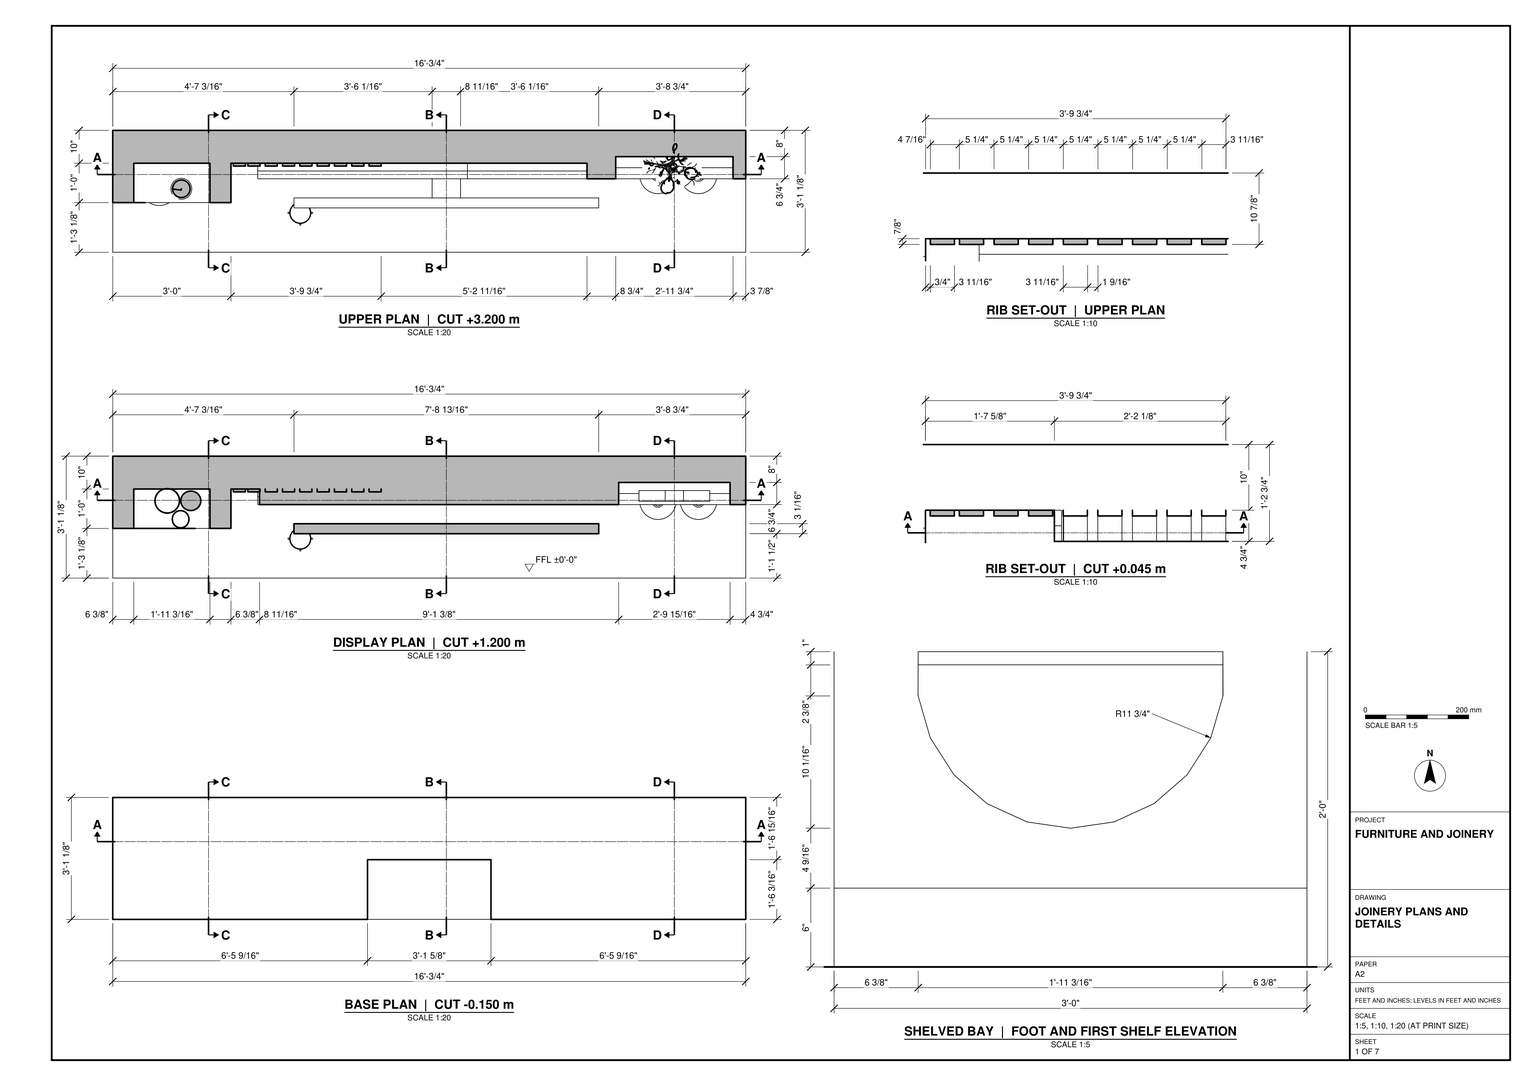
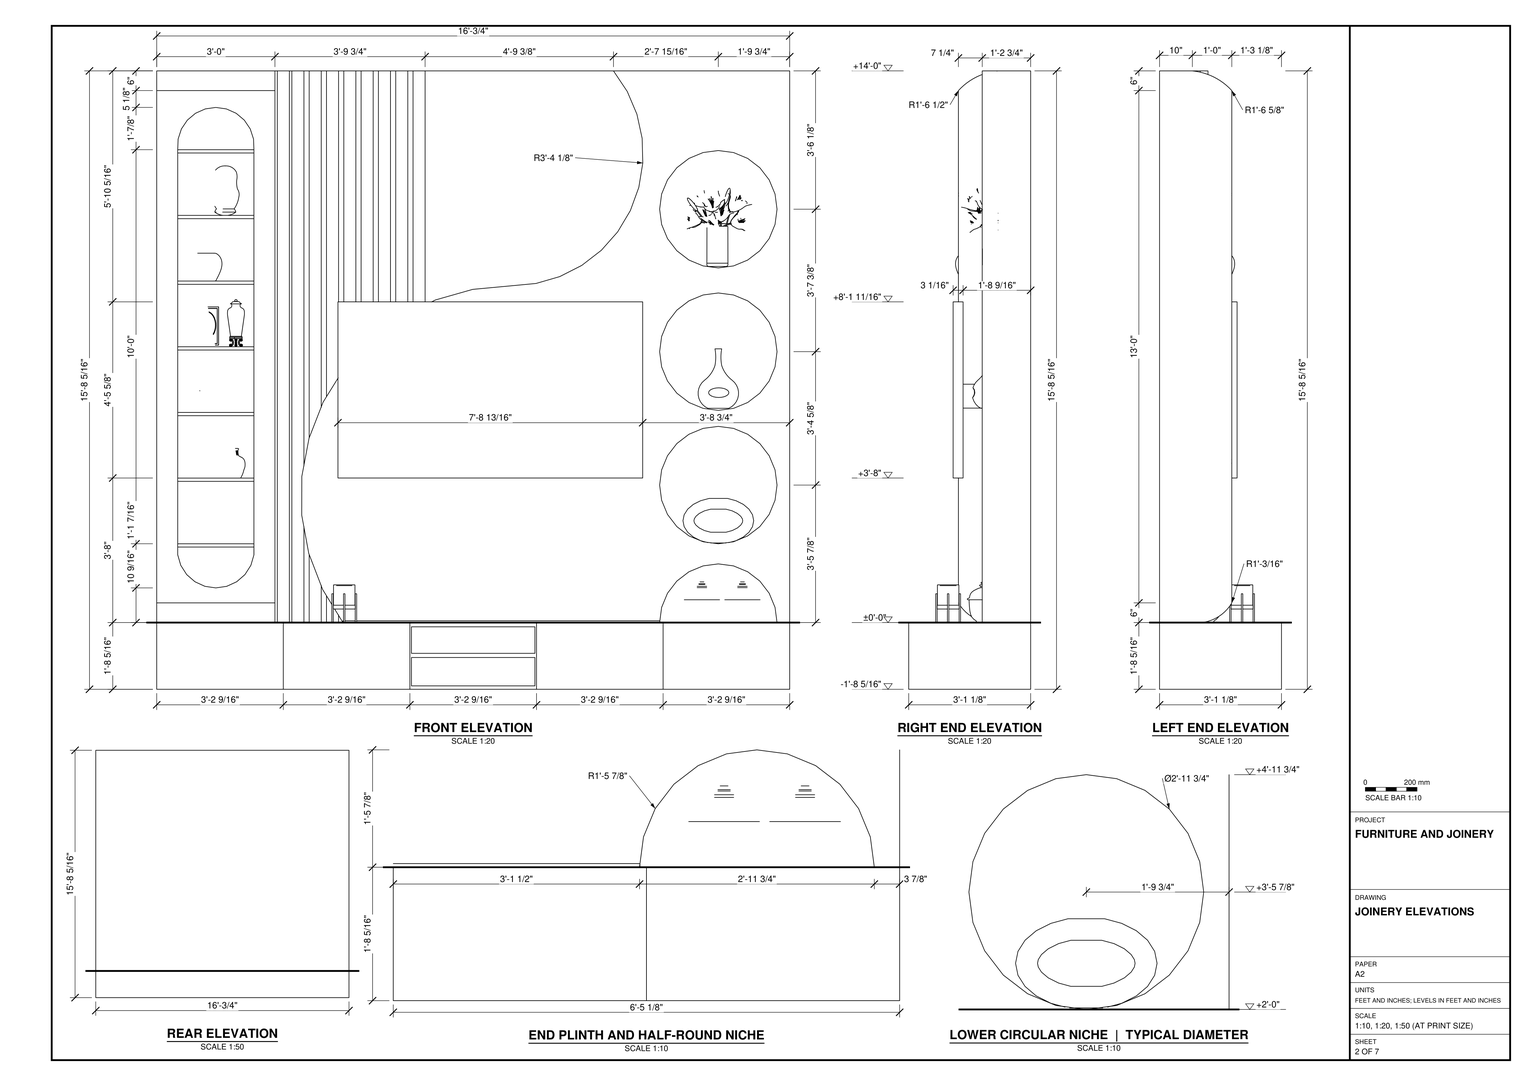
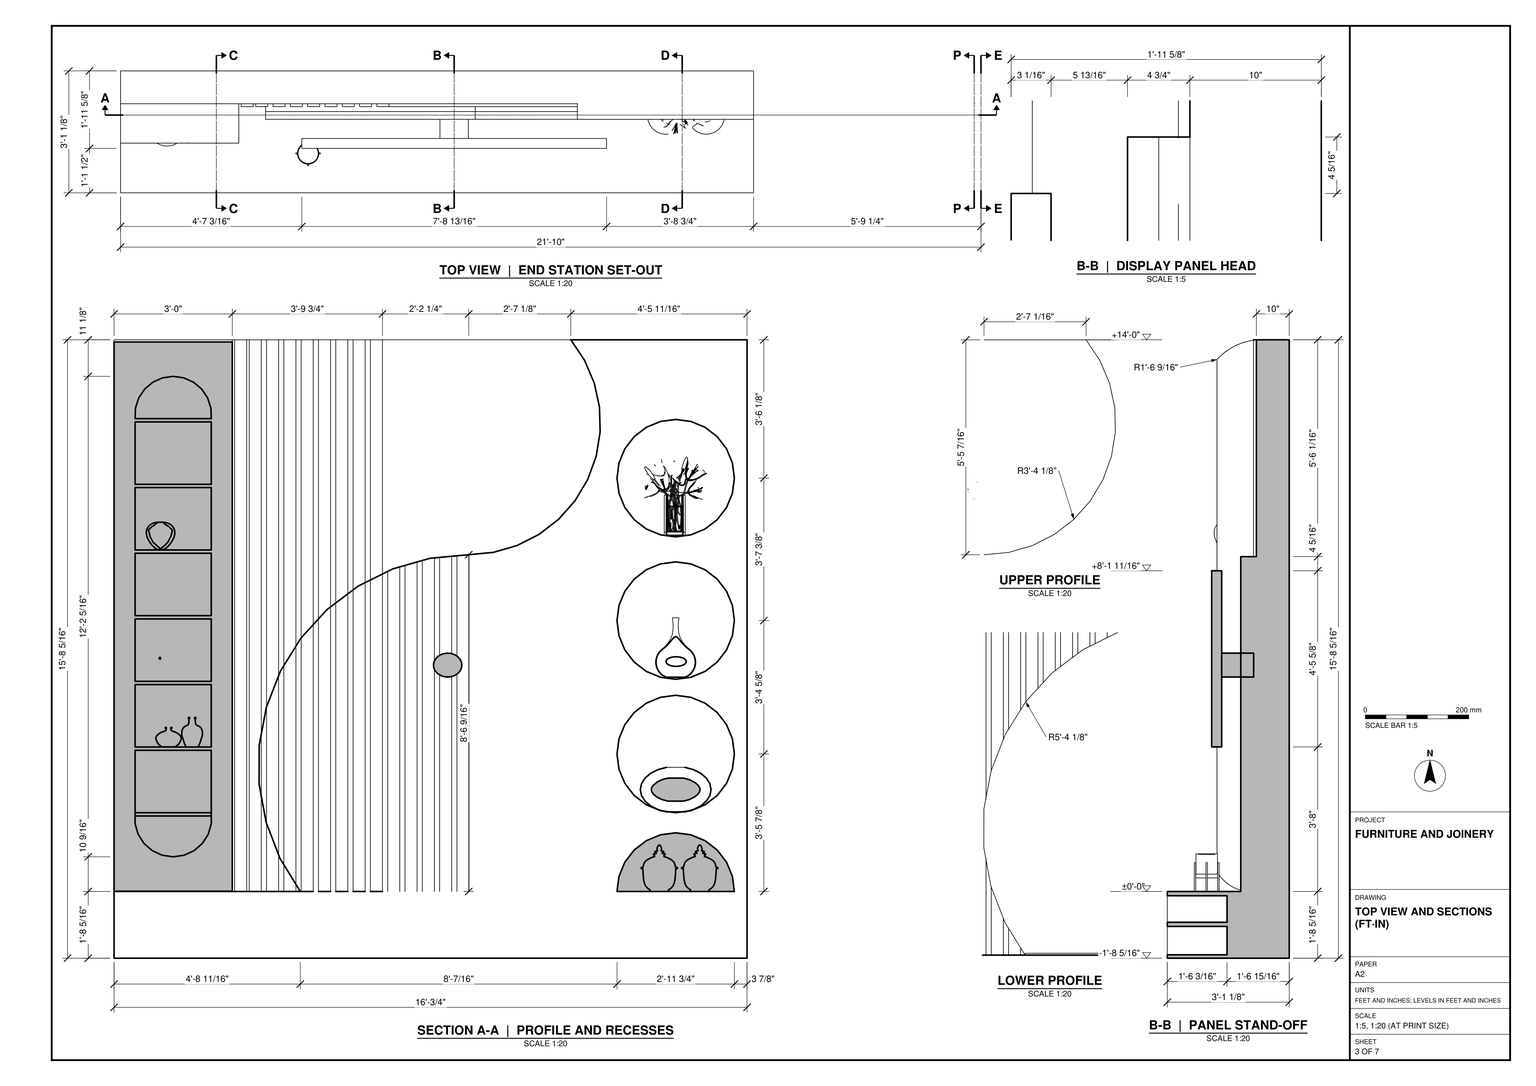
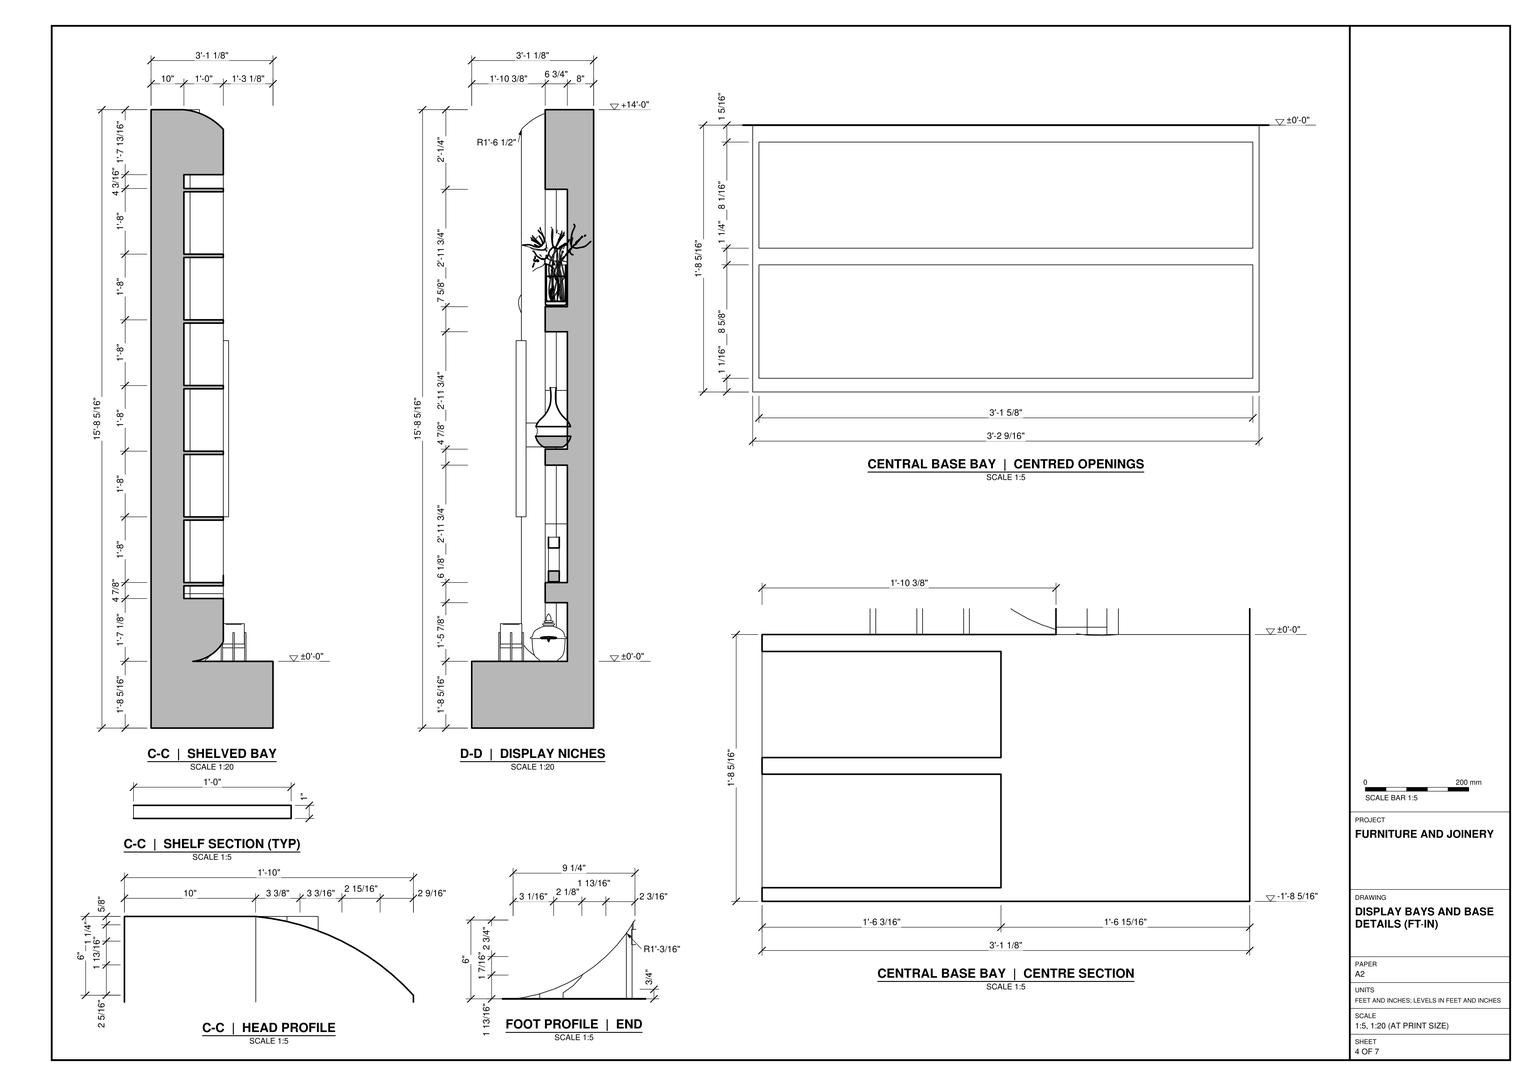
Build the display wall in SketchUp from task_files/diagram_01.pdf. Work in feet and inches. Follow the top-view end-station set-out: the overall span is 21'-10", but the joinery body itself is 16'-3/4" wide. The overall depth is 3'-1 1/8" and the overall height is 15'-8 5/16". Use ±0'-0" as the datum at the top of the plinth, with the base at -1'-8 5/16" and the wall head at +14'-0".

Form the plinth with the central setback shown in plan and the two stacked fronts shown in elevation. At the left, build the tall shelved bay with rounded ends to its opening. Beside it, model the individual vertical ribs, following the rib set-out in plan and the sweeping boundary between the ribbed and smooth faces in section A-A. Mount the rectangular display panel in front of this surface, leaving the stand-off visible in section B-B. At the right, form three circular display recesses above a half-round recess that meets the plinth. Follow the plans and sections for recess depths, backing thicknesses and end profiles.

Decor and loose items in the shelves and niches may be any suitable library components. Keep the joinery pieces in separate groups or components and use components for repeated parts. Save one SketchUp model as output_files/ribbed_display_wall_with_shelving_and_recessed_niches.skp.

# SketchUp Ruby script. Lengths in inches.
U = 1.inch
M = Sketchup.active_model
def pt(a) = Geom::Point3d.new(a.map { |v| v * U })
def face(e, loops, mat)
  f = e.add_face(loops[0].map { |a| pt(a) })
  loops[1..].each { |l| e.add_face(l.map { |a| pt(a) }).erase! }
  f.material = f.back_material = mat if mat
  f
end
# faces: each face lists its corners as indices into pts; further lists are holes
def faces(e, pts, list, mat = nil) = list.each { |f| face(e, (f[0].is_a?(Array) ? f : [f]).map { |l| l.map { |i| pts[i] } }, mat) }
# xy, xz, yz: faces in a plane at the given z, y or x. An outline is a flat list of corners, or four numbers for a rectangle; further outlines are holes
def ring(l) = l.size == 4 ? [[l[0], l[1]], [l[2], l[1]], [l[2], l[3]], [l[0], l[3]]] : l.each_slice(2).to_a
def flat(e, list, mat, &to3) = list.each { |f| face(e, (f[0].is_a?(Array) ? f : [f]).map { |l| ring(l).map { |u, v| to3.(u, v) } }, mat) }
def xy(e, z, list, mat = nil) = flat(e, list, mat) { |x, y| [x, y, z] }
def xz(e, y, list, mat = nil) = flat(e, list, mat) { |x, z| [x, y, z] }
def yz(e, x, list, mat = nil) = flat(e, list, mat) { |y, z| [x, y, z] }
def lines(e, pts, list) = list.each { |a, b| e.add_line(pt(pts[a]), pt(pts[b])) }
# prism: a flat outline (further loops are holes) pulled along v
def prism(e, loops, v, mat = nil)
  f = face(e, loops, mat); d = Geom::Vector3d.new(v.map { |x| x * U })
  f.pushpull(f.normal.samedirection?(d) ? d.length : -d.length)
end
def box(e, o, s, mat = nil) = prism(e, [[o, [o[0] + s[0], o[1], o[2]], [o[0] + s[0], o[1] + s[1], o[2]], [o[0], o[1] + s[1], o[2]]]], [0, 0, s[2]], mat)
def at(x, y, z, deg = 0) = Geom::Transformation.translation(pt([x, y, z])) * Geom::Transformation.rotation(ORIGIN, Z_AXIS, deg.degrees)
def axes(o, x, y, z) = Geom::Transformation.new([*x, 0, *y, 0, *z, 0, *pt(o).to_a, 1])
def part(name) = M.definitions.add(name)
# library, detail: a bought-in or finely detailed component or shape, given as its bounding box
def library(name, o, s) = part(name).tap { |d| box(d.entities, o, s) }
def detail(e, o, s) = box(e.add_group.entities, o, s)
def put(e, d, t, mat = nil) = e.add_instance(d, t).tap { |i| i.material = mat if mat }
def group(e, t, mat = nil) = e.add_group.tap { |g| g.transformation = t; g.material = mat if mat }.entities
root = M.entities
M.materials.add("CUEVE TILE").color = [204, 198, 186]
M.materials.add("Emissive").color = [255, 255, 255]
M.materials.add("NETFLEX TEXTURE").color = [73, 67, 67]
M.materials.add("WALL TILE").color = [226, 214, 203]
M.materials.add("WHITE WOOD TEXTURE FOR CABIN").color = [208, 209, 205]
M.materials.add("WOOD TEXTURE").color = [111, 66, 36]
M.materials.add("[Leather Red Brown]").color = [76, 40, 8]
M.materials.add("[Slate Light Tile]").color = [54, 54, 54]
c1 = library("skp5FE5",[-20.25,-9.09,-9.95],[33.36,28.86,33.4])
c2 = library("skp86D6",[-3.15,-10.14,-7.26],[20.14,20.18,14.98])
c3 = library("Lidded urn",[0,0,0],[20.74,20.74,57.81])
c4 = library("Lily Flower",[-11.23,-7.61,-0.93],[19.43,20.89,23.03])
c5 = library("KARE 65351 Vase Hole Alu Bottle ( Vase Hole Alu Bottle )",[-6.15,-1.29,0],[12.3,2.58,18.11])
c6 = part("KARE 64859 Vase Hole Alu Length ( Vase Hole Alu Quer )")
xy(c6.entities,0.2,[[-2.34,0,2.34,2.76]])
xy(c6.entities,2.96,[[-1.98,0,1.98,2.76]])
xy(c6.entities,8.85,[[-1.98,0,1.98,2.76]])
xz(c6.entities,0,[[[-2.34,0.2,2.34,0.2,4.53,0.79,6.4,1.73,7.84,2.95,8.75,4.38,9.06,5.91,8.75,7.43,7.84,8.86,6.4,10.08,4.53,11.02,2.34,11.61,-2.34,11.61,-4.53,11.02,-6.4,10.08,-7.84,8.86,-8.75,7.43,-9.06,5.91,-8.75,4.38,-7.84,2.95,-6.4,1.73,-4.53,0.79],[-1.98,2.96,-3.54,3.38,-4.87,4.05,-5.74,4.78,-6.15,5.42,-6.24,5.91,-6.15,6.39,-5.74,7.03,-4.87,7.77,-3.54,8.43,-1.98,8.85,1.98,8.85,3.54,8.43,4.87,7.77,5.74,7.03,6.15,6.39,6.24,5.91,6.15,5.42,5.74,4.78,4.87,4.05,3.54,3.38,1.98,2.96]]])
xz(c6.entities,2.76,[[[-2.34,0.2,-4.53,0.79,-6.4,1.73,-7.84,2.95,-8.75,4.38,-9.06,5.91,-8.75,7.43,-7.84,8.86,-6.4,10.08,-4.53,11.02,-2.34,11.61,2.34,11.61,4.53,11.02,6.4,10.08,7.84,8.86,8.75,7.43,9.06,5.91,8.75,4.38,7.84,2.95,6.4,1.73,4.53,0.79,2.34,0.2],[-1.98,2.96,1.98,2.96,3.54,3.38,4.87,4.05,5.74,4.78,6.15,5.42,6.24,5.91,6.15,6.39,5.74,7.03,4.87,7.77,3.54,8.43,1.98,8.85,-1.98,8.85,-3.54,8.43,-4.87,7.77,-5.74,7.03,-6.15,6.39,-6.24,5.91,-6.15,5.42,-5.74,4.78,-4.87,4.05,-3.54,3.38]]])
p = [[-2.34,0,0.2],[-4.53,0,0.79],[-4.53,2.76,0.79],[-2.34,2.76,0.2],[4.53,0,0.79],[2.34,0,0.2],
  [2.34,2.76,0.2],[4.53,2.76,0.79],[-6.4,0,1.73],[-6.4,2.76,1.73],[6.4,0,1.73],[6.4,2.76,1.73],
  [-7.84,0,2.95],[-7.84,2.76,2.95],[7.84,0,2.95],[7.84,2.76,2.95],[-8.75,0,4.38],[-8.75,2.76,4.38],
  [-3.54,0,3.38],[-1.98,0,2.96],[-1.98,2.76,2.96],[-3.54,2.76,3.38],[1.98,0,2.96],[3.54,0,3.38],
  [3.54,2.76,3.38],[1.98,2.76,2.96],[8.75,0,4.38],[8.75,2.76,4.38],[-4.87,0,4.05],[-4.87,2.76,4.05],
  [4.87,0,4.05],[4.87,2.76,4.05],[-5.74,0,4.78],[-5.74,2.76,4.78],[5.74,0,4.78],[5.74,2.76,4.78],
  [-9.06,0,5.91],[-9.06,2.76,5.91],[9.06,0,5.91],[9.06,2.76,5.91],[-6.15,0,5.42],[-6.15,2.76,5.42],
  [6.15,0,5.42],[6.15,2.76,5.42],[-6.24,0,5.91],[-6.24,2.76,5.91],[6.24,0,5.91],[6.24,2.76,5.91],
  [-8.75,0,7.43],[-8.75,2.76,7.43],[-6.15,0,6.39],[-6.15,2.76,6.39],[6.15,0,6.39],[6.15,2.76,6.39],
  [8.75,0,7.43],[8.75,2.76,7.43],[-5.74,0,7.03],[-5.74,2.76,7.03],[5.74,0,7.03],[5.74,2.76,7.03],
  [-4.87,0,7.77],[-4.87,2.76,7.77],[4.87,0,7.77],[4.87,2.76,7.77],[-7.84,0,8.86],[-7.84,2.76,8.86],
  [7.84,0,8.86],[7.84,2.76,8.86],[-3.54,0,8.43],[-3.54,2.76,8.43],[3.54,0,8.43],[3.54,2.76,8.43],
  [-1.98,0,8.85],[-1.98,2.76,8.85],[1.98,0,8.85],[1.98,2.76,8.85],[-6.4,0,10.08],[-6.4,2.76,10.08],
  [6.4,0,10.08],[6.4,2.76,10.08],[-4.53,0,11.02],[-4.53,2.76,11.02],[4.53,0,11.02],[4.53,2.76,11.02],
  [-2.34,0,11.61],[-2.34,2.76,11.61],[2.34,0,11.61],[2.34,2.76,11.61]]
faces(c6.entities,p,[[0,1,2,3],[4,5,6,7],[1,8,9,2],[10,4,7,11],[8,12,13,9],[14,10,11,15],[12,16,17,13],[18,19,20,21],
  [22,23,24,25],[26,14,15,27],[28,18,21,29],[23,30,31,24],[32,28,29,33],[30,34,35,31],[16,36,37,17],[38,26,27,39],
  [40,32,33,41],[34,42,43,35],[44,40,41,45],[42,46,47,43],[36,48,49,37],[50,44,45,51],[46,52,53,47],[54,38,39,55],
  [56,50,51,57],[52,58,59,53],[60,56,57,61],[58,62,63,59],[48,64,65,49],[66,54,55,67],[68,60,61,69],[62,70,71,63],
  [72,68,69,73],[70,74,75,71],[64,76,77,65],[78,66,67,79],[76,80,81,77],[82,78,79,83],[80,84,85,81],[86,82,83,87]])
c7 = library("Round rod",[0,0,-7.4375],[0.79,0.79,15.85])
c8 = library("Group\#146",[0,-0.5,0],[88.93,67.1,78.21])
c9 = library("Grouper\#4",[0,0,0],[24.95,24.95,44.57])
c10 = library("Group\#59",[0,0,0],[106.43,33.58,160.42])
c11 = library("Group\#22",[0,0,0],[8.59,8.59,11.1875])
c12 = library("Group\#17",[0,0,-0.5],[11.77,11.77,11.2])
xy(root,-20.3125,[[0,4.407,192.75,37.125]])
xy(root,-20.3125,[[0,0,192.75,4.407]],"Emissive")
xy(root,-19.273,[[77.577,0,115.173,18.1875]],"WHITE WOOD TEXTURE FOR CABIN")
xy(root,-10.633,[[77.577,0,115.173,18.1875]],"WHITE WOOD TEXTURE FOR CABIN")
xy(root,-9.367,[[77.577,0,115.173,18.1875]],"WHITE WOOD TEXTURE FOR CABIN")
xy(root,-1.289,[[77.577,0,115.173,18.1875]],"WHITE WOOD TEXTURE FOR CABIN")
xy(root,0,[[56.97,22.375,60.645,26.25],[62.241,22.375,65.916,26.25],[67.512,22.375,71.187,26.25],[72.783,22.375,76.458,26.25],[78.054,22.375,81.728,26.25],
  [36.72,26.25,40.395,27.125],[41.158,26.25,44.833,27.125],[46.429,26.25,50.103,27.125],[51.699,26.25,55.374,27.125]])
xy(root,0,[[0,0,192.75,0,192.75,22.375,188.89,22.375,188.89,29.125,153.14,29.125,153.14,22.375,56.718,22.375,56.718,27.125,55.374,27.125,55.374,26.25,51.699,26.25,51.699,27.125,50.103,27.125,50.103,26.25,46.429,26.25,46.429,27.125,44.833,27.125,44.833,26.25,41.158,26.25,41.158,27.125,40.395,27.125,40.395,26.25,36.72,26.25,36.72,27.125,36,27.125,36,24.402,0,24.402]],"WHITE WOOD TEXTURE FOR CABIN")
xy(root,23,[[6.401,15.125,29.599,27.125]],"WOOD TEXTURE")
xy(root,24,[[6.401,15.125,29.599,27.125]],"WOOD TEXTURE")
xy(root,43,[[6.401,15.125,29.599,27.125]],"WOOD TEXTURE")
xy(root,44,[[6.401,15.125,29.599,27.125]],"WOOD TEXTURE")
xy(root,63,[[6.401,15.125,29.599,27.125]],"WOOD TEXTURE")
xy(root,64,[[6.401,15.125,29.599,27.125]],"WOOD TEXTURE")
xy(root,83,[[6.401,15.125,29.599,27.125]],"WOOD TEXTURE")
xy(root,84,[[6.401,15.125,29.599,27.125]],"WOOD TEXTURE")
xy(root,103,[[6.401,15.125,29.599,27.125]],"WOOD TEXTURE")
xy(root,104,[[6.401,15.125,29.599,27.125]],"WOOD TEXTURE")
xy(root,123,[[6.401,15.125,29.599,27.125]],"WOOD TEXTURE")
xy(root,124,[[6.401,15.125,29.599,27.125]],"WOOD TEXTURE")
xy(root,143,[[6.401,15.125,29.599,27.125]],"WOOD TEXTURE")
xy(root,144,[[6.401,15.125,29.599,27.125]],"WOOD TEXTURE")
xy(root,168,[[139.092,22.375,192.75,22.375,192.75,37.125,0,37.125,0,27.125,139.092,27.125],[36.72,26.25,40.395,27.125],[41.158,26.25,44.833,27.125],[46.429,26.25,50.103,27.125],[51.699,26.25,55.374,27.125],
  [56.97,26.25,60.645,27.125],[62.241,26.25,65.916,27.125],[67.512,26.25,71.187,27.125],[72.783,26.25,76.458,27.125],[78.054,26.25,81.728,27.125]])
xy(root,168,[[81.728,26.25,139.092,27.125]],"Emissive")
xz(root,0,[[0,-20.3125,38.55,0],[38.55,-20.3125,77.1,0],[[77.1,-20.3125,115.65,0],[77.577,-19.273,115.173,-10.633],[77.577,-9.367,115.173,-1.289]],[115.65,-20.3125,154.2,0],[154.2,-20.3125,192.75,0]],"WHITE WOOD TEXTURE FOR CABIN")
xz(root,15.125,[[[0,6,36,162],[18,10.5625,14.69,11.04,11.649,12.432,9.125,14.626,7.323,17.444,6.401,20.615,6.39,20.655,6.401,24,6.401,144,6.516,147.243,7.52,150.329,9.336,153.019,11.822,155.104,14.786,156.424,18,156.875,21.214,156.424,24.178,155.104,26.664,153.019,28.48,150.329,29.484,147.243,29.599,144,29.599,24,29.61,20.655,29.599,20.615,28.677,17.444,26.875,14.626,24.351,12.432,21.31,11.04],[6.401,23,29.599,24]],[6.401,23,29.599,24],[6.401,43,29.599,44],[6.401,63,29.599,64],[6.401,83,29.599,84],
  [6.401,103,29.599,104],[6.401,123,29.599,124],[6.401,143,29.599,144]],"WOOD TEXTURE")
xz(root,18.1875,[[77.577,-19.273,115.173,-10.633]])
xz(root,18.1875,[[77.577,-9.367,115.173,-1.289]],"WHITE WOOD TEXTURE FOR CABIN")
xz(root,22.375,[[153.14,0,153.213,0,153.213,0.558]])
xz(root,22.375,[[56.718,0,153.14,0,153.213,0.558,56.718,0.558]],"Emissive")
xz(root,22.375,[[[56.718,0,56.718,0.558,153.213,0.558,153.749,4.626,155.535,8.9375,158.375,12.64,162.077,15.48,166.388,17.266,171.015,17.875,175.641,17.266,179.952,15.48,183.654,12.64,186.495,8.9375,188.281,4.626,188.89,0,192.75,0,192.75,168,139.092,168,143.276,161.747,146.219,154.823,147.817,147.471,148.013,139.95,146.801,132.525,144.224,125.456,140.372,118.993,135.381,113.364,129.426,108.766,122.717,105.36,115.49,103.268,108,102.5625,96.239,101.474,84.877,98.247,74.3,92.989,64.867,85.88,56.899,77.161,50.666,67.128,46.379,56.122,44.185,44.516,44.157,32.704,46.297,21.088,50.532,10.062],[171.015,108,166.388,108.609,162.077,110.395,158.375,113.235,155.535,116.9375,153.749,121.249,153.14,125.875,153.749,130.501,155.535,134.8125,158.375,138.515,162.077,141.355,166.388,143.141,171.015,143.75,175.641,143.141,179.952,141.355,183.654,138.515,186.495,134.8125,188.281,130.501,188.89,125.875,188.281,121.249,186.495,116.9375,183.654,113.235,179.952,110.395,175.641,108.609],[171.015,64.625,166.388,65.234,162.077,67.02,158.375,69.86,155.535,73.5625,153.749,77.874,153.14,82.5,153.749,87.126,155.535,91.4375,158.375,95.14,162.077,97.98,166.388,99.766,171.015,100.375,175.641,99.766,179.952,97.98,183.654,95.14,186.495,91.4375,188.281,87.126,188.89,82.5,188.281,77.874,186.495,73.5625,183.654,69.86,179.952,67.02,175.641,65.234],[171.015,24,166.388,24.609,162.077,26.395,158.375,29.235,155.535,32.9375,153.749,37.249,153.14,41.875,153.749,46.501,155.535,50.8125,158.375,54.515,162.077,57.355,166.388,59.141,171.015,59.75,175.641,59.141,179.952,57.355,183.654,54.515,186.495,50.8125,188.281,46.501,188.89,41.875,188.281,37.249,186.495,32.9375,183.654,29.235,179.952,26.395,175.641,24.609]]],"WALL TILE")
xz(root,26.25,[[36.72,0,40.395,168],[41.158,0,44.833,168],[46.429,0,50.103,168],[51.699,0,55.374,168],[56.97,0,60.645,168],
  [62.241,0,65.916,168],[67.512,0,71.187,168],[72.783,0,76.458,168],[78.054,0,81.728,168]],"WOOD TEXTURE")
xz(root,27.125,[[36.72,0,40.395,168],[41.158,0,44.833,0,44.833,29.038,44.157,32.704,44.185,44.516,44.833,47.942,44.833,168,41.158,168],[44.833,0,46.429,0,46.429,20.746,46.297,21.088,44.833,29.038],[46.429,0,50.103,0,50.103,11.178,46.429,20.746],[50.103,0,51.699,0,51.699,8.163,50.532,10.062,50.103,11.178],
  [51.699,0,55.374,0,55.374,2.186,51.699,8.163],[55.374,0,56.718,0,55.374,2.186],[6.401,20.615,6.401,24,6.39,20.655],[29.599,20.615,29.61,20.655,29.599,24],[46.429,56.249,50.103,65.684,50.103,168,46.429,168],
  [51.699,68.792,55.374,74.707,55.374,168,51.699,168],[56.97,77.239,60.645,81.26,60.645,168,56.97,168],[62.241,83.007,64.867,85.88,65.916,86.67,65.916,168,62.241,168],[67.512,87.873,71.187,90.643,71.187,168,67.512,168],[72.783,91.846,74.3,92.989,76.458,94.062,76.458,168,72.783,168],
  [78.054,94.855,81.728,96.682,81.728,168,78.054,168]])
xz(root,27.125,[[81.728,96.682,83.324,97.475,84.877,98.247,86.999,98.85,88.595,99.303,92.27,100.347,93.866,100.8,96.239,101.474,97.541,101.595,99.137,101.742,102.812,102.082,104.408,102.23,108,102.5625,108.083,102.57,115.49,103.268,122.717,105.36,129.426,108.766,135.381,113.364,140.372,118.993,144.224,125.456,146.801,132.525,148.013,139.95,147.817,147.471,146.219,154.823,143.276,161.747,139.092,168,81.728,168]],"CUEVE TILE")
xz(root,27.125,[[36,0,36.72,168],[40.395,0,41.158,168],[44.833,47.942,46.379,56.122,46.429,56.249,46.429,168,44.833,168],[50.103,65.684,50.666,67.128,51.699,68.792,51.699,168,50.103,168],[55.374,74.707,56.899,77.161,56.97,77.239,56.97,168,55.374,168],
  [60.645,81.26,62.241,83.007,62.241,168,60.645,168],[65.916,86.67,67.512,87.873,67.512,168,65.916,168],[71.187,90.643,72.783,91.846,72.783,168,71.187,168],[76.458,94.062,78.054,94.855,78.054,168,76.458,168]],"Emissive")
xz(root,27.125,[[18,10.5625,21.31,11.04,24.351,12.432,26.875,14.626,28.677,17.444,29.599,20.615,29.599,23,6.401,23,6.401,20.615,7.323,17.444,9.125,14.626,11.649,12.432,14.69,11.04],[6.401,24,29.599,43],[6.401,44,29.599,63],[6.401,64,29.599,83],[6.401,84,29.599,103],
  [6.401,104,29.599,123],[6.401,124,29.599,143],[6.401,144,29.599,144,29.484,147.243,28.48,150.329,26.664,153.019,24.178,155.104,21.214,156.424,18,156.875,14.786,156.424,11.822,155.104,9.336,153.019,7.52,150.329,6.516,147.243]],"WOOD TEXTURE")
xz(root,27.21,[[261.938,119.54,262,119.54,261.93,119.542]])
xz(root,29.125,[[153.14,0,188.89,0,188.281,4.626,186.495,8.9375,183.654,12.64,179.952,15.48,175.641,17.266,171.015,17.875,166.388,17.266,162.077,15.48,158.375,12.64,155.535,8.9375,153.749,4.626],[171.015,24,175.641,24.609,179.952,26.395,183.654,29.235,186.495,32.9375,188.281,37.249,188.89,41.875,188.281,46.501,186.495,50.8125,183.654,54.515,179.952,57.355,175.641,59.141,171.015,59.75,166.388,59.141,162.077,57.355,158.375,54.515,155.535,50.8125,153.749,46.501,153.14,41.875,153.749,37.249,155.535,32.9375,158.375,29.235,162.077,26.395,166.388,24.609],[171.015,64.625,175.641,65.234,179.952,67.02,183.654,69.86,186.495,73.5625,188.281,77.874,188.89,82.5,188.281,87.126,186.495,91.4375,183.654,95.14,179.952,97.98,175.641,99.766,171.015,100.375,166.388,99.766,162.077,97.98,158.375,95.14,155.535,91.4375,153.749,87.126,153.14,82.5,153.749,77.874,155.535,73.5625,158.375,69.86,162.077,67.02,166.388,65.234],[171.015,108,175.641,108.609,179.952,110.395,183.654,113.235,186.495,116.9375,188.281,121.249,188.89,125.875,188.281,130.501,186.495,134.8125,183.654,138.515,179.952,141.355,175.641,143.141,171.015,143.75,166.388,143.141,162.077,141.355,158.375,138.515,155.535,134.8125,153.749,130.501,153.14,125.875,153.749,121.249,155.535,116.9375,158.375,113.235,162.077,110.395,166.388,108.609]],"WALL TILE")
xz(root,37.125,[[0,-20.3125,192.75,168]])
yz(root,0,[[0,-20.3125,37.125,0]],"WHITE WOOD TEXTURE FOR CABIN")
yz(root,0,[[24.402,0,23.589,0.103,22.436,0.363,21.313,0.734,20.231,1.211,19.2,1.791,18.229,2.467,17.328,3.233,16.506,4.083,15.769,5.008,15.125,6,15.125,162,15.921,162.821,16.765,163.593,17.655,164.31,18.588,164.972,19.559,165.575,20.566,166.118,21.604,166.598,22.67,167.013,23.759,167.362,24.867,167.643,25.99,167.856,27.125,168,37.125,168,37.125,0]],"WOOD TEXTURE")
yz(root,6.401,[[15.125,23,27.125,24]])
yz(root,6.401,[[25.25,24,27.125,43],[25.25,44,27.125,63],[25.25,64,27.125,83],[25.25,84,27.125,103],[25.25,104,27.125,123],
  [25.25,124,27.125,143]],"Emissive")
yz(root,6.401,[[15.125,24,25.25,43],[15.125,44,25.25,63],[15.125,64,25.25,83],[15.125,84,25.25,103],[15.125,104,25.25,123],
  [15.125,124,25.25,143]],"WOOD TEXTURE")
yz(root,29.599,[[15.125,23,27.125,24]])
yz(root,29.599,[[25.25,24,27.125,43],[25.25,44,27.125,63],[25.25,64,27.125,83],[25.25,84,27.125,103],[25.25,104,27.125,123],
  [25.25,124,27.125,143]],"Emissive")
yz(root,29.599,[[15.125,24,25.25,43],[15.125,44,25.25,63],[15.125,64,25.25,83],[15.125,84,25.25,103],[15.125,104,25.25,123],
  [15.125,124,25.25,143]],"WOOD TEXTURE")
yz(root,36,[[25.945,-0.08,27.125,0,24.402,0,24.763,-0.046]])
yz(root,36,[[24.402,0,27.125,0,27.125,168,25.99,167.856,24.867,167.643,23.759,167.362,22.67,167.013,21.604,166.598,20.566,166.118,19.559,165.575,18.588,164.972,17.655,164.31,16.765,163.593,15.921,162.821,15.125,162,15.125,6,15.769,5.008,16.506,4.083,17.328,3.233,18.229,2.467,19.2,1.791,20.231,1.211,21.313,0.734,22.436,0.363,23.589,0.103]],"WOOD TEXTURE")
yz(root,36.72,[[26.25,0,27.125,168]])
yz(root,40.395,[[26.25,0,27.125,168]])
yz(root,41.158,[[26.25,0,27.125,168]])
yz(root,44.833,[[26.25,0,27.125,168]])
yz(root,46.429,[[26.25,0,27.125,168]])
yz(root,50.103,[[26.25,0,27.125,168]])
yz(root,51.699,[[26.25,0,27.125,168]])
yz(root,55.374,[[26.25,0,27.125,168]])
yz(root,56.97,[[26.25,0,27.125,168]])
yz(root,60.645,[[26.25,0,27.125,168]])
yz(root,62.241,[[26.25,0,27.125,168]])
yz(root,65.916,[[26.25,0,27.125,168]])
yz(root,67.512,[[26.25,0,27.125,168]])
yz(root,71.187,[[26.25,0,27.125,168]])
yz(root,72.783,[[26.25,0,27.125,168]])
yz(root,76.458,[[26.25,0,27.125,168]])
yz(root,77.577,[[0,-19.273,18.1875,-10.633],[0,-9.367,18.1875,-1.289]],"WHITE WOOD TEXTURE FOR CABIN")
yz(root,78.054,[[26.25,0,27.125,168]])
yz(root,81.728,[[26.25,0,27.125,168]])
yz(root,115.173,[[0,-19.273,18.1875,-10.633],[0,-9.367,18.1875,-1.289]],"WHITE WOOD TEXTURE FOR CABIN")
yz(root,192.75,[[0,-20.3125,37.125,-20.3125,37.125,168,22.375,168,22.375,0,0,0]],"WHITE WOOD TEXTURE FOR CABIN")
p = [[50.532,22.375,10.062],[50.532,24.75,10.062],[56.718,24.75,0],[56.718,22.375,0],[153.14,22.375,0],[153.14,25.75,0],
  [153.749,25.75,4.626],[153.749,22.375,4.626],[153.213,22.375,0.558],[188.281,22.375,4.626],[188.281,25.75,4.626],[188.89,25.75,0],
  [188.89,22.375,0],[36,24.402,0],[36,23.589,0.103],[0,23.589,0.103],[0,24.402,0],[56.718,27.125,0],
  [50.532,27.125,10.062],[51.699,27.125,8.163],[55.374,27.125,2.186],[153.749,29.125,4.626],[153.14,29.125,0],[188.89,29.125,0],
  [188.281,29.125,4.626],[36,22.436,0.363],[0,22.436,0.363],[36,21.313,0.734],[0,21.313,0.734],[36,20.231,1.211],
  [0,20.231,1.211],[36,19.2,1.791],[0,19.2,1.791],[36,18.229,2.467],[0,18.229,2.467],[36,17.328,3.233],
  [0,17.328,3.233],[36,16.506,4.083],[0,16.506,4.083],[36,15.769,5.008],[0,15.769,5.008],[155.535,25.75,8.9375],
  [155.535,22.375,8.9375],[186.495,22.375,8.9375],[186.495,25.75,8.9375],[155.535,29.125,8.9375],[186.495,29.125,8.9375],[36,15.125,6],
  [0,15.125,6],[158.375,25.75,12.64],[158.375,22.375,12.64],[183.654,22.375,12.64],[183.654,25.75,12.64],[158.375,29.125,12.64],
  [183.654,29.125,12.64],[46.297,22.375,21.088],[46.297,24.75,21.088],[46.297,27.125,21.088],[46.429,27.125,20.746],[50.103,27.125,11.178],
  [18,15.125,10.5625],[18,25.25,10.5625],[14.69,25.25,11.04],[14.69,15.125,11.04],[21.31,15.125,11.04],[21.31,25.25,11.04],
  [14.69,27.125,11.04],[18,27.125,10.5625],[21.31,27.125,11.04],[11.649,25.25,12.432],[11.649,15.125,12.432],[24.351,15.125,12.432],
  [24.351,25.25,12.432],[11.649,27.125,12.432],[24.351,27.125,12.432],[9.125,25.25,14.626],[9.125,15.125,14.626],[26.875,15.125,14.626],
  [26.875,25.25,14.626],[9.125,27.125,14.626],[26.875,27.125,14.626],[162.077,25.75,15.48],[162.077,22.375,15.48],[179.952,22.375,15.48],
  [179.952,25.75,15.48],[162.077,29.125,15.48],[179.952,29.125,15.48],[7.323,25.25,17.444],[7.323,15.125,17.444],[28.677,15.125,17.444],
  [28.677,25.25,17.444],[7.323,27.125,17.444],[28.677,27.125,17.444],[166.388,25.75,17.266],[166.388,22.375,17.266],[175.641,22.375,17.266],
  [175.641,25.75,17.266],[166.388,29.125,17.266],[175.641,29.125,17.266],[171.015,25.75,17.875],[171.015,22.375,17.875],[171.015,29.125,17.875],
  [6.401,25.25,20.615],[6.401,15.125,20.615],[29.599,15.125,20.615],[29.599,25.25,20.615],[6.401,27.125,20.615],[29.599,27.125,20.615],
  [6.39,25.25,20.655],[6.39,15.125,20.655],[29.61,15.125,20.655],[29.61,25.25,20.655],[6.39,27.125,20.655],[29.61,27.125,20.655],
  [6.401,25.25,24],[6.401,15.125,24],[29.599,15.125,24],[29.599,25.25,24],[6.401,27.125,24],[29.599,27.125,24],
  [44.157,22.375,32.704],[44.157,24.75,32.704],[44.157,27.125,32.704],[44.833,27.125,29.038],[171.015,22.375,24],[171.015,25.75,24],
  [166.388,25.75,24.609],[166.388,22.375,24.609],[175.641,22.375,24.609],[175.641,25.75,24.609],[166.388,29.125,24.609],[171.015,29.125,24],
  [175.641,29.125,24.609],[162.077,25.75,26.395],[162.077,22.375,26.395],[179.952,22.375,26.395],[179.952,25.75,26.395],[162.077,29.125,26.395],
  [179.952,29.125,26.395],[158.375,25.75,29.235],[158.375,22.375,29.235],[183.654,22.375,29.235],[183.654,25.75,29.235],[158.375,29.125,29.235],
  [183.654,29.125,29.235],[155.535,25.75,32.9375],[155.535,22.375,32.9375],[186.495,22.375,32.9375],[186.495,25.75,32.9375],[186.495,29.125,32.9375],
  [155.535,29.125,32.9375],[44.185,22.375,44.516],[44.185,24.75,44.516],[44.185,27.125,44.516],[153.749,25.75,37.249],[153.749,22.375,37.249],
  [188.281,22.375,37.249],[188.281,25.75,37.249],[188.281,29.125,37.249],[153.749,29.125,37.249],[153.14,25.75,41.875],[153.14,22.375,41.875],
  [188.89,22.375,41.875],[188.89,25.75,41.875],[188.89,29.125,41.875],[153.14,29.125,41.875],[153.749,25.75,46.501],[153.749,22.375,46.501],
  [188.281,22.375,46.501],[188.281,25.75,46.501],[188.281,29.125,46.501],[153.749,29.125,46.501],[46.379,22.375,56.122],[46.379,24.75,56.122],
  [46.379,27.125,56.122],[44.833,27.125,47.942],[155.535,25.75,50.8125],[155.535,22.375,50.8125],[186.495,22.375,50.8125],[186.495,25.75,50.8125],
  [186.495,29.125,50.8125],[155.535,29.125,50.8125],[158.375,25.75,54.515],[158.375,22.375,54.515],[183.654,22.375,54.515],[183.654,25.75,54.515],
  [183.654,29.125,54.515],[158.375,29.125,54.515],[162.077,25.75,57.355],[162.077,22.375,57.355],[179.952,22.375,57.355],[179.952,25.75,57.355],
  [162.077,29.125,57.355],[179.952,29.125,57.355],[50.666,22.375,67.128],[50.666,24.75,67.128],[50.666,27.125,67.128],[50.103,27.125,65.684],
  [46.429,27.125,56.249],[166.388,25.75,59.141],[166.388,22.375,59.141],[175.641,22.375,59.141],[175.641,25.75,59.141],[166.388,29.125,59.141],
  [175.641,29.125,59.141],[171.015,25.75,59.75],[171.015,22.375,59.75],[171.015,29.125,59.75],[171.015,22.375,64.625],[171.015,25.75,64.625],
  [166.388,25.75,65.234],[166.388,22.375,65.234],[175.641,22.375,65.234],[175.641,25.75,65.234],[166.388,29.125,65.234],[171.015,29.125,64.625],
  [175.641,29.125,65.234],[162.077,25.75,67.02],[162.077,22.375,67.02],[179.952,22.375,67.02],[179.952,25.75,67.02],[162.077,29.125,67.02],
  [179.952,29.125,67.02],[158.375,25.75,69.86],[158.375,22.375,69.86],[183.654,22.375,69.86],[183.654,25.75,69.86],[158.375,29.125,69.86],
  [183.654,29.125,69.86],[56.899,22.375,77.161],[56.899,24.75,77.161],[56.899,27.125,77.161],[55.374,27.125,74.707],[51.699,27.125,68.792],
  [155.535,25.75,73.5625],[155.535,22.375,73.5625],[186.495,22.375,73.5625],[186.495,25.75,73.5625],[155.535,29.125,73.5625],[186.495,29.125,73.5625],
  [153.749,25.75,77.874],[153.749,22.375,77.874],[188.281,22.375,77.874],[188.281,25.75,77.874],[153.749,29.125,77.874],[188.281,29.125,77.874],
  [64.867,22.375,85.88],[64.867,24.75,85.88],[64.867,27.125,85.88],[62.241,27.125,83.007],[60.645,27.125,81.26],[56.97,27.125,77.239],
  [153.14,25.75,82.5],[153.14,22.375,82.5],[188.89,22.375,82.5],[188.89,25.75,82.5],[153.14,29.125,82.5],[188.89,29.125,82.5],
  [153.749,25.75,87.126],[153.749,22.375,87.126],[188.281,22.375,87.126],[188.281,25.75,87.126],[153.749,29.125,87.126],[188.281,29.125,87.126],
  [74.3,22.375,92.989],[74.3,24.75,92.989],[74.3,27.125,92.989],[72.783,27.125,91.846],[71.187,27.125,90.643],[67.512,27.125,87.873],
  [65.916,27.125,86.67],[155.535,25.75,91.4375],[155.535,22.375,91.4375],[186.495,22.375,91.4375],[186.495,25.75,91.4375],[155.535,29.125,91.4375],
  [186.495,29.125,91.4375],[158.375,25.75,95.14],[158.375,22.375,95.14],[183.654,22.375,95.14],[183.654,25.75,95.14],[158.375,29.125,95.14],
  [183.654,29.125,95.14],[84.877,22.375,98.247],[84.877,24.75,98.247],[84.877,27.125,98.247],[83.324,27.125,97.475],[81.728,27.125,96.682],
  [78.054,27.125,94.855],[76.458,27.125,94.062],[162.077,25.75,97.98],[162.077,22.375,97.98],[179.952,22.375,97.98],[179.952,25.75,97.98],
  [162.077,29.125,97.98],[179.952,29.125,97.98],[166.388,25.75,99.766],[166.388,22.375,99.766],[175.641,22.375,99.766],[175.641,25.75,99.766],
  [166.388,29.125,99.766],[175.641,29.125,99.766],[96.239,22.375,101.474],[96.239,24.75,101.474],[96.239,27.125,101.474],[93.866,27.125,100.8],
  [92.27,27.125,100.347],[88.595,27.125,99.303],[86.999,27.125,98.85],[171.015,25.75,100.375],[171.015,22.375,100.375],[171.015,29.125,100.375],
  [108,22.375,102.5625],[108,24.75,102.5625],[108,27.125,102.5625],[104.408,27.125,102.23],[102.812,27.125,102.082],[99.137,27.125,101.742],
  [97.541,27.125,101.595],[115.49,22.375,103.268],[115.49,24.75,103.268],[115.49,27.125,103.268],[108.083,27.125,102.57],[122.717,22.375,105.36],
  [122.717,24.75,105.36],[122.717,27.125,105.36],[129.426,22.375,108.766],[129.426,24.75,108.766],[129.426,27.125,108.766],[171.015,22.375,108],
  [171.015,25.75,108],[166.388,25.75,108.609],[166.388,22.375,108.609],[175.641,22.375,108.609],[175.641,25.75,108.609],[166.388,29.125,108.609],
  [171.015,29.125,108],[175.641,29.125,108.609],[162.077,25.75,110.395],[162.077,22.375,110.395],[179.952,22.375,110.395],[179.952,25.75,110.395],
  [162.077,29.125,110.395],[179.952,29.125,110.395],[135.381,22.375,113.364],[135.381,24.75,113.364],[135.381,27.125,113.364],[158.375,25.75,113.235],
  [158.375,22.375,113.235],[183.654,22.375,113.235],[183.654,25.75,113.235],[158.375,29.125,113.235],[183.654,29.125,113.235],[155.535,25.75,116.9375],
  [155.535,22.375,116.9375],[186.495,22.375,116.9375],[186.495,25.75,116.9375],[186.495,29.125,116.9375],[155.535,29.125,116.9375],[140.372,22.375,118.993],
  [140.372,24.75,118.993],[140.372,27.125,118.993],[153.749,25.75,121.249],[153.749,22.375,121.249],[188.281,22.375,121.249],[188.281,25.75,121.249],
  [188.281,29.125,121.249],[153.749,29.125,121.249],[144.224,22.375,125.456],[144.224,24.75,125.456],[144.224,27.125,125.456],[153.14,25.75,125.875],
  [153.14,22.375,125.875],[188.89,22.375,125.875],[188.89,25.75,125.875],[188.89,29.125,125.875],[153.14,29.125,125.875],[146.801,22.375,132.525],
  [146.801,24.75,132.525],[146.801,27.125,132.525],[153.749,25.75,130.501],[153.749,22.375,130.501],[188.281,22.375,130.501],[188.281,25.75,130.501],
  [188.281,29.125,130.501],[153.749,29.125,130.501],[155.535,25.75,134.8125],[155.535,22.375,134.8125],[186.495,22.375,134.8125],[186.495,25.75,134.8125],
  [186.495,29.125,134.8125],[155.535,29.125,134.8125],[148.013,22.375,139.95],[148.013,24.75,139.95],[148.013,27.125,139.95],[158.375,25.75,138.515],
  [158.375,22.375,138.515],[183.654,22.375,138.515],[183.654,25.75,138.515],[183.654,29.125,138.515],[158.375,29.125,138.515],[162.077,25.75,141.355],
  [162.077,22.375,141.355],[179.952,22.375,141.355],[179.952,25.75,141.355],[162.077,29.125,141.355],[179.952,29.125,141.355],[147.817,22.375,147.471],
  [147.817,24.75,147.471],[147.817,27.125,147.471],[166.388,25.75,143.141],[166.388,22.375,143.141],[175.641,22.375,143.141],[175.641,25.75,143.141],
  [166.388,29.125,143.141],[175.641,29.125,143.141],[171.015,25.75,143.75],[171.015,22.375,143.75],[171.015,29.125,143.75],[6.401,15.125,144],
  [6.401,25.25,144],[6.516,25.25,147.243],[6.516,15.125,147.243],[29.484,15.125,147.243],[29.484,25.25,147.243],[29.599,25.25,144],
  [29.599,15.125,144],[6.516,27.125,147.243],[6.401,27.125,144],[29.599,27.125,144],[29.484,27.125,147.243],[7.52,25.25,150.329],
  [7.52,15.125,150.329],[28.48,15.125,150.329],[28.48,25.25,150.329],[7.52,27.125,150.329],[28.48,27.125,150.329],[146.219,22.375,154.823],
  [146.219,24.75,154.823],[146.219,27.125,154.823],[9.336,25.25,153.019],[9.336,15.125,153.019],[26.664,15.125,153.019],[26.664,25.25,153.019],
  [9.336,27.125,153.019],[26.664,27.125,153.019],[11.822,25.25,155.104],[11.822,15.125,155.104],[24.178,15.125,155.104],[24.178,25.25,155.104],
  [11.822,27.125,155.104],[24.178,27.125,155.104],[143.276,22.375,161.747],[143.276,24.75,161.747],[143.276,27.125,161.747],[14.786,25.25,156.424],
  [14.786,15.125,156.424],[21.214,15.125,156.424],[21.214,25.25,156.424],[14.786,27.125,156.424],[21.214,27.125,156.424],[18,25.25,156.875],
  [18,15.125,156.875],[18,27.125,156.875],[139.092,22.375,168],[139.092,24.75,168],[139.092,26.25,168],[139.092,27.125,168],
  [36,15.125,162],[36,15.921,162.821],[0,15.921,162.821],[0,15.125,162],[36,16.765,163.593],[0,16.765,163.593],
  [36,17.655,164.31],[0,17.655,164.31],[36,18.588,164.972],[0,18.588,164.972],[36,19.559,165.575],[0,19.559,165.575],
  [36,20.566,166.118],[0,20.566,166.118],[36,21.604,166.598],[0,21.604,166.598],[36,22.67,167.013],[0,22.67,167.013],
  [36,23.759,167.362],[0,23.759,167.362],[36,24.867,167.643],[0,24.867,167.643],[36,25.99,167.856],[0,25.99,167.856],
  [36,27.125,168],[0,27.125,168],[86.999,27.125,29.038],[86.999,27.125,0],[86.999,27.125,47.942],[83.324,27.125,0],
  [92.27,27.125,29.038],[92.27,27.125,0],[92.27,27.125,47.942],[88.595,27.125,0],[97.541,27.125,29.038],[97.541,27.125,0],
  [97.541,27.125,47.942],[93.866,27.125,0],[102.812,27.125,29.038],[102.812,27.125,0],[102.812,27.125,47.942],[99.137,27.125,0],
  [104.408,27.125,0],[104.408,26.25,0],[108.083,27.125,0],[108.083,26.25,0],[108.083,27.125,29.038],[108.083,27.125,47.942],
  [262.768,27.21,124.659],[262.768,27.21,124.673],[259.929,27.21,122.542],[260.023,27.21,122.38],[260.023,27.21,122.542],[260.097,27.21,122.441],
  [260.023,27.21,122.334],[260.097,27.21,122.395],[260.019,27.21,121.713],[260.019,27.21,121.716],[57.044,26.25,0.558],[57.044,22.375,0.558]]
faces(root,p,[[0,1,2,3],[4,5,6,7,8],[9,10,11,12],[7,6,41,42],[43,44,10,9],[42,41,49,50],[51,52,44,43],[55,56,1,0],
  [50,49,81,82],[83,84,52,51],[82,81,93,94],[95,96,84,83],[94,93,99,100],[100,99,96,95],[120,121,56,55],[124,125,126,127],
  [128,129,125,124],[127,126,133,134],[135,136,129,128],[134,133,139,140],[141,142,136,135],[140,139,145,146],[147,148,142,141],[151,152,121,120],
  [146,145,154,155],[156,157,148,147],[155,154,160,161],[162,163,157,156],[161,160,166,167],[168,169,163,162],[172,173,152,151],[167,166,176,177],
  [178,179,169,168],[177,176,182,183],[184,185,179,178],[183,182,188,189],[190,191,185,184],[194,195,173,172],[189,188,199,200],[201,202,191,190],
  [200,199,205,206],[206,205,202,201],[208,209,210,211],[212,213,209,208],[211,210,217,218],[219,220,213,212],[218,217,223,224],[225,226,220,219],
  [229,230,195,194],[224,223,234,235],[236,237,226,225],[235,234,240,241],[242,243,237,236],[246,247,230,229],[241,240,252,253],[254,255,243,242],
  [253,252,258,259],[260,261,255,254],[264,265,247,246],[259,258,271,272],[273,274,261,260],[272,271,277,278],[279,280,274,273],[283,284,265,264],
  [278,277,290,291],[292,293,280,279],[291,290,296,297],[298,299,293,292],[302,303,284,283],[297,296,309,310],[310,309,299,298],[312,313,303,302],
  [319,320,313,312],[323,324,320,319],[326,327,324,323],[329,330,331,332],[333,334,330,329],[332,331,338,339],[340,341,334,333],[344,345,327,326],
  [339,338,347,348],[349,350,341,340],[348,347,353,354],[355,356,350,349],[359,360,345,344],[354,353,362,363],[364,365,356,355],[368,369,360,359],
  [363,362,371,372],[373,374,365,364],[377,378,369,368],[372,371,380,381],[382,383,374,373],[381,380,386,387],[388,389,383,382],[392,393,378,377],
  [387,386,395,396],[397,398,389,388],[396,395,401,402],[403,404,398,397],[407,408,393,392],[402,401,410,411],[412,413,404,403],[411,410,416,417],
  [417,416,413,412],[437,438,408,407],[452,453,438,437],[464,465,453,452]],"WALL TILE")
faces(root,p,[[13,14,15,16],[14,25,26,15],[25,27,28,26],[27,29,30,28],[29,31,32,30],[31,33,34,32],[33,35,36,34],[35,37,38,36],
  [37,39,40,38],[39,47,48,40],[60,61,62,63],[64,65,61,60],[63,62,69,70],[71,72,65,64],[70,69,75,76],[77,78,72,71],
  [76,75,87,88],[89,90,78,77],[88,87,102,103],[104,105,90,89],[103,102,108,109],[110,111,105,104],[109,108,114,115],[116,117,111,110],
  [419,420,421,422],[423,424,425,426],[422,421,431,432],[433,434,424,423],[432,431,440,441],[442,443,434,433],[441,440,446,447],[448,449,443,442],
  [447,446,455,456],[457,458,449,448],[456,455,461,462],[462,461,458,457],[468,469,470,471],[469,472,473,470],[472,474,475,473],[474,476,477,475],
  [476,478,479,477],[478,480,481,479],[480,482,483,481],[482,484,485,483],[484,486,487,485],[486,488,489,487],[488,490,491,489],[490,492,493,491]],"WOOD TEXTURE")
faces(root,p,[[17,2,1,18,19,20],[21,6,5,22],[23,11,10,24],[45,41,6,21],[24,10,44,46],[53,49,41,45],[46,44,52,54],[18,1,56,57,58,59],
  [66,62,61,67],[67,61,65,68],[73,69,62,66],[68,65,72,74],[79,75,69,73],[74,72,78,80],[85,81,49,53],[54,52,84,86],
  [91,87,75,79],[80,78,90,92],[97,93,81,85],[86,84,96,98],[101,99,93,97],[98,96,99,101],[106,102,87,91],[92,90,105,107],
  [112,108,102,106],[107,105,111,113],[118,114,108,112],[113,111,117,119],[57,56,121,122,123],[130,126,125,131],[131,125,129,132],[137,133,126,130],
  [132,129,136,138],[143,139,133,137],[138,136,142,144],[144,142,148,149],[150,145,139,143],[122,121,152,153],[149,148,157,158],[159,154,145,150],
  [158,157,163,164],[165,160,154,159],[164,163,169,170],[171,166,160,165],[153,152,173,174,175],[170,169,179,180],[181,176,166,171],[180,179,185,186],
  [187,182,176,181],[192,188,182,187],[186,185,191,193],[174,173,195,196,197,198],[203,199,188,192],[193,191,202,204],[207,205,199,203],[204,202,205,207],
  [214,210,209,215],[215,209,213,216],[221,217,210,214],[216,213,220,222],[227,223,217,221],[222,220,226,228],[196,195,230,231,232,233],[238,234,223,227],
  [228,226,237,239],[244,240,234,238],[239,237,243,245],[231,230,247,248,249,250,251],[256,252,240,244],[245,243,255,257],[262,258,252,256],[257,255,261,263],
  [248,247,265,266,267,268,269,270],[275,271,258,262],[263,261,274,276],[281,277,271,275],[276,274,280,282],[266,265,284,285,286,287,288,289],[294,290,277,281],[282,280,293,295],
  [300,296,290,294],[295,293,299,301],[285,284,303,304,305,306,307,308],[311,309,296,300],[301,299,309,311],[304,303,313,314,315,316,317,318],[314,313,320,321,322],[321,320,324,325],
  [325,324,327,328],[335,331,330,336],[336,330,334,337],[342,338,331,335],[337,334,341,343],[328,327,345,346],[351,347,338,342],[343,341,350,352],
  [352,350,356,357],[358,353,347,351],[346,345,360,361],[357,356,365,366],[367,362,353,358],[361,360,369,370],[366,365,374,375],[376,371,362,367],
  [370,369,378,379],[375,374,383,384],[385,380,371,376],[384,383,389,390],[391,386,380,385],[379,378,393,394],[390,389,398,399],[400,395,386,391],
  [405,401,395,400],[399,398,404,406],[394,393,408,409],[414,410,401,405],[406,404,413,415],[418,416,410,414],[415,413,416,418],[427,421,420,428],
  [429,425,424,430],[435,431,421,427],[430,424,434,436],[409,408,438,439],[444,440,431,435],[436,434,443,445],[450,446,440,444],[445,443,449,451],
  [439,438,453,454],[459,455,446,450],[451,449,458,460],[463,461,455,459],[460,458,461,463],[454,453,465,466,467]],"Emissive")
lines(root,p,[[494,495],[496,494],[286,497],[308,496],[498,499],[500,498],[307,501],[306,500],[502,503],[504,502],[305,505],[318,504],
  [506,507],[508,506],[317,509],[316,508],[510,511],[512,513],[514,512],[515,514],[315,510],[322,515],[516,517],[518,519],
  [518,520],[520,521],[522,523],[523,521],[519,522],[524,525],[526,527]])
put(root,c1,axes([18.3,23.54,48.24],[-0.4256,0,0],[0,-0.4256,0],[0,0,0.4256]))
put(root,c2,axes([18.08,19.9375,108.11],[-0.5664,0,0],[0,-0.5664,0],[0,0,0.5664]))
put(root,c3,axes([26.72,22.56,84],[-0.2494,0,0],[0,-0.2494,0],[0,0,0.2494]))
put(root,c4,axes([172.88,23.24,109.44],[1.0723,0,0],[0,1.0723,0],[0,0,1.0723]))
put(root,c5,axes([171.01,24.82,65.25],[1,0,0],[0,4.1728,0],[0,0,1]))
put(root,c6,axes([171.01,23.375,24],[1.18968,0,0],[0,1.18968,0],[0,0,1.18968]))
put(root,c7,axes([57.32,15.78,4.125],[-0.55471,0,0],[0,-0.55471,0],[0,0,0.55471]),"[Slate Light Tile]")
put(root,c7,axes([60.89,11.78,4.125],[0,0.55471,0],[-0.55471,0,0],[0,0,0.55471]))
put(root,c7,axes([53.32,12.22,4.125],[0,-0.55471,0],[0.55471,0,0],[0,0,0.55471]))
put(root,c7,axes([56.89,8.22,4.125],[0.55471,0,0],[0,0.55471,0],[0,0,0.55471]))
put(root,c8,axes([20.9,24.09,64],[-0.13456,0,0],[0,-0.13456,0],[0,0,0.13456]))
put(root,c9,axes([25.11,23.57,124],[-0.33833,0,0],[0,-0.33833,0],[0,0,0.33833]))
put(root,c10,axes([10.73,19.36,84.47],[0.06888,0.02366,0],[0.02366,-0.06888,0],[0,0,0.07283]))
put(root,c11,axes([160.44,17.83,0],[1.2987,0,0],[0,1.2987,0],[0,0,1.2987]))
put(root,c11,axes([172.77,17.83,0],[1.2987,0,0],[0,1.2987,0],[0,0,1.2987]))
g1 = group(root,at(55.1875,11.14,44.02))
prism(g1,[[[42.21,15.16,23.98],[42.09,15.16,24.75],[42.07,15.16,24.92],[42.21,15.16,25.86],[42.65,15.16,26.74],[43.34,15.16,27.5],[44.23,15.16,28.07],[45.28,15.16,28.4375],[46.4,15.16,28.5625],[47.52,15.16,28.4375],[48.5625,15.16,28.07],[49.46,15.16,27.5],[50.15,15.16,26.74],[50.58,15.16,25.86],[50.7,15.16,25.1],[50.73,15.16,24.92],[50.58,15.16,23.98],[50.15,15.16,23.1],[49.46,15.16,22.35],[48.5625,15.16,21.77],[47.52,15.16,21.41],[46.4,15.16,21.29],[45.28,15.16,21.41],[44.23,15.16,21.77],[43.34,15.16,22.35],[42.65,15.16,23.1]]],[0,-9.74,0])
g2 = group(g1,at(0,0,0))
xy(g2,0,[[0,2.375,92.8,5.41]])
xy(g2,53.65,[[0,2.375,92.8,5.41]])
xz(g2,2.375,[[0,0,92.8,53.65]],"NETFLEX TEXTURE")
xz(g2,5.41,[[0,0,92.8,53.65]])
yz(g2,0,[[2.375,0,5.41,53.65]])
yz(g2,92.8,[[2.375,0,5.41,53.65]])
put(root,c12,axes([53.84,8.74,5.5625],[0.55471,0,0],[0,0.55471,0],[0,0,0.55471]),"[Leather Red Brown]")
g3 = group(root,at(53.73,8.63,4.125))
prism(g3,[[[3.28,6.75,0],[3.46,6.75,0],[3.46,3.46,0],[6.75,3.46,0],[6.75,3.26,0],[3.48,3.26,0],[3.48,0,0],[3.26,0,0],[3.26,3.26,0],[0,3.26,0],[0,3.46,0],[3.28,3.46,0]]],[0,0,1.16],"[Slate Light Tile]")
